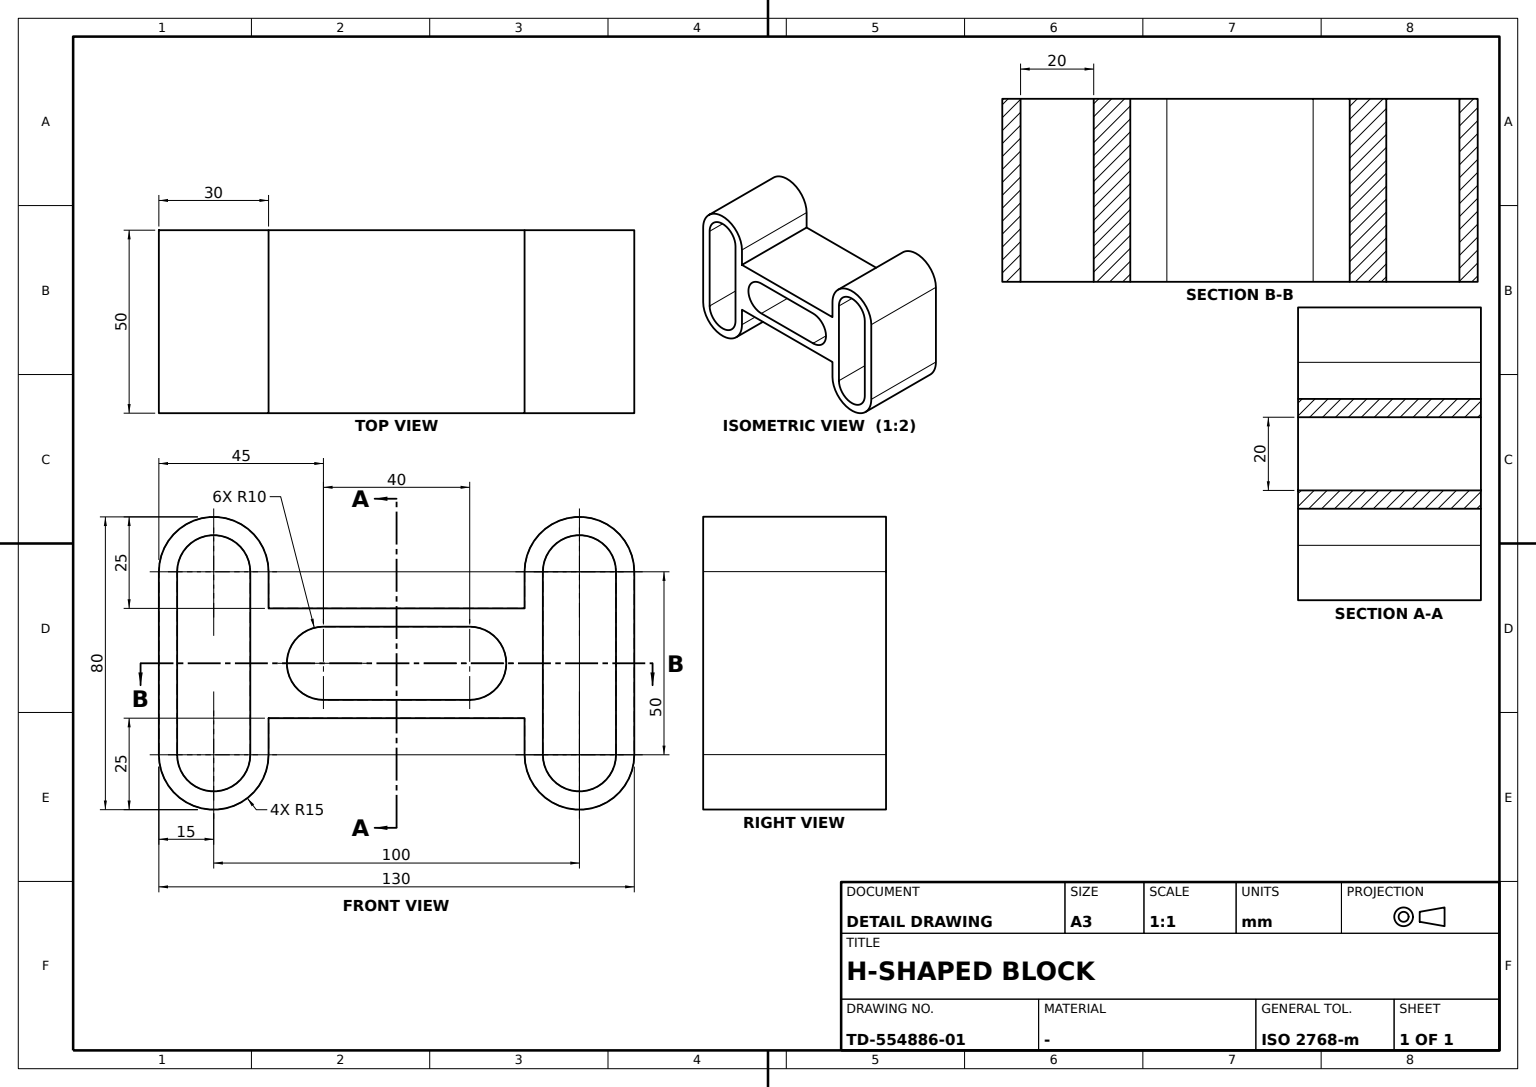
ISO-10303-21;
HEADER;
FILE_DESCRIPTION((''),'2;1');
FILE_NAME('','',(''),(''),'','','');
FILE_SCHEMA(('AUTOMOTIVE_DESIGN'));
ENDSEC;
DATA;
#1=APPLICATION_CONTEXT('');
#2=PRODUCT_CONTEXT('',#1,'mechanical');
#3=PRODUCT('','','',(#2));
#4=PRODUCT_DEFINITION_FORMATION('','',#3);
#5=PRODUCT_DEFINITION_CONTEXT('',#1,'design');
#6=PRODUCT_DEFINITION('','',#4,#5);
#7=PRODUCT_DEFINITION_SHAPE('','',#6);
#8=(LENGTH_UNIT()NAMED_UNIT(*)SI_UNIT(.MILLI.,.METRE.));
#9=(NAMED_UNIT(*)PLANE_ANGLE_UNIT()SI_UNIT($,.RADIAN.));
#10=(NAMED_UNIT(*)SI_UNIT($,.STERADIAN.)SOLID_ANGLE_UNIT());
#11=UNCERTAINTY_MEASURE_WITH_UNIT(LENGTH_MEASURE(1.E-05),#8,'distance_accuracy_value','');
#12=(GEOMETRIC_REPRESENTATION_CONTEXT(3)GLOBAL_UNCERTAINTY_ASSIGNED_CONTEXT((#11))GLOBAL_UNIT_ASSIGNED_CONTEXT((#8,#9,#10))REPRESENTATION_CONTEXT('',''));
#13=CARTESIAN_POINT('',(-25.,30.,0.));
#14=VERTEX_POINT('',#13);
#15=CARTESIAN_POINT('',(-25.,20.,10.));
#16=VERTEX_POINT('',#15);
#17=CARTESIAN_POINT('',(-25.,20.,0.));
#18=DIRECTION('',(1.,0.,0.));
#19=DIRECTION('',(0.,1.,0.));
#20=AXIS2_PLACEMENT_3D('',#17,#18,#19);
#21=CIRCLE('',#20,10.);
#22=EDGE_CURVE('',#14,#16,#21,.T.);
#23=ORIENTED_EDGE('',*,*,#22,.F.);
#24=CARTESIAN_POINT('',(25.,30.,0.));
#25=VERTEX_POINT('',#24);
#26=CARTESIAN_POINT('',(0.,30.,0.));
#27=DIRECTION('',(-1.,0.,0.));
#28=VECTOR('',#27,1000.);
#29=LINE('',#26,#28);
#30=EDGE_CURVE('',#25,#14,#29,.T.);
#31=ORIENTED_EDGE('',*,*,#30,.F.);
#32=CARTESIAN_POINT('',(25.,20.,10.));
#33=VERTEX_POINT('',#32);
#34=CARTESIAN_POINT('',(25.,20.,0.));
#35=AXIS2_PLACEMENT_3D('',#34,#18,#19);
#36=CIRCLE('',#35,10.);
#37=EDGE_CURVE('',#25,#33,#36,.T.);
#38=ORIENTED_EDGE('',*,*,#37,.T.);
#39=CARTESIAN_POINT('',(0.,20.,10.));
#40=LINE('',#39,#28);
#41=EDGE_CURVE('',#33,#16,#40,.T.);
#42=ORIENTED_EDGE('',*,*,#41,.T.);
#43=EDGE_LOOP('',(#23,#31,#38,#42));
#44=FACE_OUTER_BOUND('',#43,.T.);
#45=CARTESIAN_POINT('',(0.,20.,0.));
#46=AXIS2_PLACEMENT_3D('',#45,#27,#19);
#47=CYLINDRICAL_SURFACE('',#46,10.);
#48=ADVANCED_FACE('',(#44),#47,.F.);
#49=CARTESIAN_POINT('',(-25.,-35.,15.));
#50=VERTEX_POINT('',#49);
#51=CARTESIAN_POINT('',(25.,-35.,15.));
#52=VERTEX_POINT('',#51);
#53=CARTESIAN_POINT('',(0.,-35.,15.));
#54=VECTOR('',#18,1000.);
#55=LINE('',#53,#54);
#56=EDGE_CURVE('',#50,#52,#55,.T.);
#57=ORIENTED_EDGE('',*,*,#56,.T.);
#58=CARTESIAN_POINT('',(25.,35.,15.));
#59=VERTEX_POINT('',#58);
#60=CARTESIAN_POINT('',(25.,0.,15.));
#61=DIRECTION('',(0.,-1.,0.));
#62=VECTOR('',#61,1000.);
#63=LINE('',#60,#62);
#64=EDGE_CURVE('',#59,#52,#63,.T.);
#65=ORIENTED_EDGE('',*,*,#64,.F.);
#66=CARTESIAN_POINT('',(-25.,35.,15.));
#67=VERTEX_POINT('',#66);
#68=CARTESIAN_POINT('',(0.,35.,15.));
#69=LINE('',#68,#54);
#70=EDGE_CURVE('',#67,#59,#69,.T.);
#71=ORIENTED_EDGE('',*,*,#70,.F.);
#72=CARTESIAN_POINT('',(-25.,0.,15.));
#73=LINE('',#72,#62);
#74=EDGE_CURVE('',#67,#50,#73,.T.);
#75=ORIENTED_EDGE('',*,*,#74,.T.);
#76=EDGE_LOOP('',(#57,#65,#71,#75));
#77=FACE_OUTER_BOUND('',#76,.T.);
#78=DIRECTION('',(0.,0.,-1.));
#79=AXIS2_PLACEMENT_3D('',#53,#78,#19);
#80=PLANE('',#79);
#81=ADVANCED_FACE('',(#77),#80,.F.);
#82=CARTESIAN_POINT('',(25.,-20.,10.));
#83=VERTEX_POINT('',#82);
#84=CARTESIAN_POINT('',(25.,0.,10.));
#85=LINE('',#84,#62);
#86=EDGE_CURVE('',#33,#83,#85,.T.);
#87=ORIENTED_EDGE('',*,*,#86,.T.);
#88=CARTESIAN_POINT('',(-25.,-20.,10.));
#89=VERTEX_POINT('',#88);
#90=CARTESIAN_POINT('',(0.,-20.,10.));
#91=LINE('',#90,#28);
#92=EDGE_CURVE('',#83,#89,#91,.T.);
#93=ORIENTED_EDGE('',*,*,#92,.T.);
#94=CARTESIAN_POINT('',(-25.,0.,10.));
#95=LINE('',#94,#62);
#96=EDGE_CURVE('',#16,#89,#95,.T.);
#97=ORIENTED_EDGE('',*,*,#96,.F.);
#98=ORIENTED_EDGE('',*,*,#41,.F.);
#99=EDGE_LOOP('',(#87,#93,#97,#98));
#100=FACE_OUTER_BOUND('',#99,.T.);
#101=DIRECTION('',(0.,0.,1.));
#102=AXIS2_PLACEMENT_3D('',#90,#101,#19);
#103=PLANE('',#102);
#104=ADVANCED_FACE('',(#100),#103,.F.);
#105=CARTESIAN_POINT('',(25.,-20.,-10.));
#106=VERTEX_POINT('',#105);
#107=CARTESIAN_POINT('',(25.,20.,-10.));
#108=VERTEX_POINT('',#107);
#109=CARTESIAN_POINT('',(25.,0.,-10.));
#110=VECTOR('',#19,1000.);
#111=LINE('',#109,#110);
#112=EDGE_CURVE('',#106,#108,#111,.T.);
#113=ORIENTED_EDGE('',*,*,#112,.T.);
#114=CARTESIAN_POINT('',(-25.,20.,-10.));
#115=VERTEX_POINT('',#114);
#116=CARTESIAN_POINT('',(0.,20.,-10.));
#117=LINE('',#116,#28);
#118=EDGE_CURVE('',#108,#115,#117,.T.);
#119=ORIENTED_EDGE('',*,*,#118,.T.);
#120=CARTESIAN_POINT('',(-25.,-20.,-10.));
#121=VERTEX_POINT('',#120);
#122=CARTESIAN_POINT('',(-25.,0.,-10.));
#123=LINE('',#122,#110);
#124=EDGE_CURVE('',#121,#115,#123,.T.);
#125=ORIENTED_EDGE('',*,*,#124,.F.);
#126=CARTESIAN_POINT('',(0.,-20.,-10.));
#127=LINE('',#126,#28);
#128=EDGE_CURVE('',#106,#121,#127,.T.);
#129=ORIENTED_EDGE('',*,*,#128,.F.);
#130=EDGE_LOOP('',(#113,#119,#125,#129));
#131=FACE_OUTER_BOUND('',#130,.T.);
#132=AXIS2_PLACEMENT_3D('',#116,#78,#61);
#133=PLANE('',#132);
#134=ADVANCED_FACE('',(#131),#133,.F.);
#135=CARTESIAN_POINT('',(25.,65.,25.));
#136=VERTEX_POINT('',#135);
#137=CARTESIAN_POINT('',(25.,35.,25.));
#138=VERTEX_POINT('',#137);
#139=CARTESIAN_POINT('',(25.,50.,25.));
#140=AXIS2_PLACEMENT_3D('',#139,#18,#19);
#141=CIRCLE('',#140,15.);
#142=EDGE_CURVE('',#136,#138,#141,.T.);
#143=ORIENTED_EDGE('',*,*,#142,.F.);
#144=CARTESIAN_POINT('',(-25.,65.,25.));
#145=VERTEX_POINT('',#144);
#146=CARTESIAN_POINT('',(0.,65.,25.));
#147=LINE('',#146,#54);
#148=EDGE_CURVE('',#145,#136,#147,.T.);
#149=ORIENTED_EDGE('',*,*,#148,.F.);
#150=CARTESIAN_POINT('',(-25.,35.,25.));
#151=VERTEX_POINT('',#150);
#152=CARTESIAN_POINT('',(-25.,50.,25.));
#153=AXIS2_PLACEMENT_3D('',#152,#18,#19);
#154=CIRCLE('',#153,15.);
#155=EDGE_CURVE('',#145,#151,#154,.T.);
#156=ORIENTED_EDGE('',*,*,#155,.T.);
#157=CARTESIAN_POINT('',(0.,35.,25.));
#158=LINE('',#157,#54);
#159=EDGE_CURVE('',#151,#138,#158,.T.);
#160=ORIENTED_EDGE('',*,*,#159,.T.);
#161=EDGE_LOOP('',(#143,#149,#156,#160));
#162=FACE_OUTER_BOUND('',#161,.T.);
#163=CARTESIAN_POINT('',(0.,50.,25.));
#164=AXIS2_PLACEMENT_3D('',#163,#27,#19);
#165=CYLINDRICAL_SURFACE('',#164,15.);
#166=ADVANCED_FACE('',(#162),#165,.T.);
#167=CARTESIAN_POINT('',(-25.,35.,-15.));
#168=VERTEX_POINT('',#167);
#169=CARTESIAN_POINT('',(25.,35.,-15.));
#170=VERTEX_POINT('',#169);
#171=CARTESIAN_POINT('',(0.,35.,-15.));
#172=LINE('',#171,#54);
#173=EDGE_CURVE('',#168,#170,#172,.T.);
#174=ORIENTED_EDGE('',*,*,#173,.F.);
#175=CARTESIAN_POINT('',(-25.,35.,-25.));
#176=VERTEX_POINT('',#175);
#177=CARTESIAN_POINT('',(-25.,35.,-20.));
#178=VECTOR('',#78,1000.);
#179=LINE('',#177,#178);
#180=EDGE_CURVE('',#168,#176,#179,.T.);
#181=ORIENTED_EDGE('',*,*,#180,.T.);
#182=CARTESIAN_POINT('',(25.,35.,-25.));
#183=VERTEX_POINT('',#182);
#184=CARTESIAN_POINT('',(0.,35.,-25.));
#185=LINE('',#184,#54);
#186=EDGE_CURVE('',#176,#183,#185,.T.);
#187=ORIENTED_EDGE('',*,*,#186,.T.);
#188=CARTESIAN_POINT('',(25.,35.,-20.));
#189=LINE('',#188,#178);
#190=EDGE_CURVE('',#170,#183,#189,.T.);
#191=ORIENTED_EDGE('',*,*,#190,.F.);
#192=EDGE_LOOP('',(#174,#181,#187,#191));
#193=FACE_OUTER_BOUND('',#192,.T.);
#194=AXIS2_PLACEMENT_3D('',#171,#61,#78);
#195=PLANE('',#194);
#196=ADVANCED_FACE('',(#193),#195,.T.);
#197=CARTESIAN_POINT('',(25.,-35.,-25.));
#198=VERTEX_POINT('',#197);
#199=CARTESIAN_POINT('',(25.,-35.,-15.));
#200=VERTEX_POINT('',#199);
#201=CARTESIAN_POINT('',(25.,-35.,-20.));
#202=VECTOR('',#101,1000.);
#203=LINE('',#201,#202);
#204=EDGE_CURVE('',#198,#200,#203,.T.);
#205=ORIENTED_EDGE('',*,*,#204,.F.);
#206=CARTESIAN_POINT('',(-25.,-35.,-25.));
#207=VERTEX_POINT('',#206);
#208=CARTESIAN_POINT('',(0.,-35.,-25.));
#209=LINE('',#208,#54);
#210=EDGE_CURVE('',#207,#198,#209,.T.);
#211=ORIENTED_EDGE('',*,*,#210,.F.);
#212=CARTESIAN_POINT('',(-25.,-35.,-15.));
#213=VERTEX_POINT('',#212);
#214=CARTESIAN_POINT('',(-25.,-35.,-20.));
#215=LINE('',#214,#202);
#216=EDGE_CURVE('',#207,#213,#215,.T.);
#217=ORIENTED_EDGE('',*,*,#216,.T.);
#218=CARTESIAN_POINT('',(0.,-35.,-15.));
#219=LINE('',#218,#54);
#220=EDGE_CURVE('',#213,#200,#219,.T.);
#221=ORIENTED_EDGE('',*,*,#220,.T.);
#222=EDGE_LOOP('',(#205,#211,#217,#221));
#223=FACE_OUTER_BOUND('',#222,.T.);
#224=AXIS2_PLACEMENT_3D('',#53,#19,#101);
#225=PLANE('',#224);
#226=ADVANCED_FACE('',(#223),#225,.T.);
#227=CARTESIAN_POINT('',(25.,65.,-25.));
#228=VERTEX_POINT('',#227);
#229=CARTESIAN_POINT('',(25.,50.,-25.));
#230=AXIS2_PLACEMENT_3D('',#229,#18,#19);
#231=CIRCLE('',#230,15.);
#232=EDGE_CURVE('',#183,#228,#231,.T.);
#233=ORIENTED_EDGE('',*,*,#232,.F.);
#234=ORIENTED_EDGE('',*,*,#186,.F.);
#235=CARTESIAN_POINT('',(-25.,65.,-25.));
#236=VERTEX_POINT('',#235);
#237=CARTESIAN_POINT('',(-25.,50.,-25.));
#238=AXIS2_PLACEMENT_3D('',#237,#18,#19);
#239=CIRCLE('',#238,15.);
#240=EDGE_CURVE('',#176,#236,#239,.T.);
#241=ORIENTED_EDGE('',*,*,#240,.T.);
#242=CARTESIAN_POINT('',(0.,65.,-25.));
#243=LINE('',#242,#54);
#244=EDGE_CURVE('',#236,#228,#243,.T.);
#245=ORIENTED_EDGE('',*,*,#244,.T.);
#246=EDGE_LOOP('',(#233,#234,#241,#245));
#247=FACE_OUTER_BOUND('',#246,.T.);
#248=CARTESIAN_POINT('',(0.,50.,-25.));
#249=AXIS2_PLACEMENT_3D('',#248,#27,#19);
#250=CYLINDRICAL_SURFACE('',#249,15.);
#251=ADVANCED_FACE('',(#247),#250,.T.);
#252=CARTESIAN_POINT('',(25.,-60.,25.));
#253=VERTEX_POINT('',#252);
#254=CARTESIAN_POINT('',(-25.,-60.,25.));
#255=VERTEX_POINT('',#254);
#256=CARTESIAN_POINT('',(0.,-60.,25.));
#257=LINE('',#256,#28);
#258=EDGE_CURVE('',#253,#255,#257,.T.);
#259=ORIENTED_EDGE('',*,*,#258,.T.);
#260=CARTESIAN_POINT('',(-25.,-40.,25.));
#261=VERTEX_POINT('',#260);
#262=CARTESIAN_POINT('',(-25.,-50.,25.));
#263=AXIS2_PLACEMENT_3D('',#262,#18,#19);
#264=CIRCLE('',#263,10.);
#265=EDGE_CURVE('',#261,#255,#264,.T.);
#266=ORIENTED_EDGE('',*,*,#265,.F.);
#267=CARTESIAN_POINT('',(25.,-40.,25.));
#268=VERTEX_POINT('',#267);
#269=CARTESIAN_POINT('',(0.,-40.,25.));
#270=LINE('',#269,#28);
#271=EDGE_CURVE('',#268,#261,#270,.T.);
#272=ORIENTED_EDGE('',*,*,#271,.F.);
#273=CARTESIAN_POINT('',(25.,-50.,25.));
#274=AXIS2_PLACEMENT_3D('',#273,#18,#19);
#275=CIRCLE('',#274,10.);
#276=EDGE_CURVE('',#268,#253,#275,.T.);
#277=ORIENTED_EDGE('',*,*,#276,.T.);
#278=EDGE_LOOP('',(#259,#266,#272,#277));
#279=FACE_OUTER_BOUND('',#278,.T.);
#280=CARTESIAN_POINT('',(0.,-50.,25.));
#281=AXIS2_PLACEMENT_3D('',#280,#27,#19);
#282=CYLINDRICAL_SURFACE('',#281,10.);
#283=ADVANCED_FACE('',(#279),#282,.F.);
#284=ORIENTED_EDGE('',*,*,#30,.T.);
#285=EDGE_CURVE('',#115,#14,#21,.T.);
#286=ORIENTED_EDGE('',*,*,#285,.F.);
#287=ORIENTED_EDGE('',*,*,#118,.F.);
#288=EDGE_CURVE('',#108,#25,#36,.T.);
#289=ORIENTED_EDGE('',*,*,#288,.T.);
#290=EDGE_LOOP('',(#284,#286,#287,#289));
#291=FACE_OUTER_BOUND('',#290,.T.);
#292=ADVANCED_FACE('',(#291),#47,.F.);
#293=CARTESIAN_POINT('',(-25.,65.,0.));
#294=LINE('',#293,#202);
#295=EDGE_CURVE('',#236,#145,#294,.T.);
#296=ORIENTED_EDGE('',*,*,#295,.T.);
#297=ORIENTED_EDGE('',*,*,#148,.T.);
#298=CARTESIAN_POINT('',(25.,65.,0.));
#299=LINE('',#298,#202);
#300=EDGE_CURVE('',#228,#136,#299,.T.);
#301=ORIENTED_EDGE('',*,*,#300,.F.);
#302=ORIENTED_EDGE('',*,*,#244,.F.);
#303=EDGE_LOOP('',(#296,#297,#301,#302));
#304=FACE_OUTER_BOUND('',#303,.T.);
#305=AXIS2_PLACEMENT_3D('',#146,#61,#78);
#306=PLANE('',#305);
#307=ADVANCED_FACE('',(#304),#306,.F.);
#308=CARTESIAN_POINT('',(-25.,-65.,-25.));
#309=VERTEX_POINT('',#308);
#310=CARTESIAN_POINT('',(25.,-65.,-25.));
#311=VERTEX_POINT('',#310);
#312=CARTESIAN_POINT('',(0.,-65.,-25.));
#313=LINE('',#312,#54);
#314=EDGE_CURVE('',#309,#311,#313,.T.);
#315=ORIENTED_EDGE('',*,*,#314,.T.);
#316=CARTESIAN_POINT('',(25.,-65.,25.));
#317=VERTEX_POINT('',#316);
#318=CARTESIAN_POINT('',(25.,-65.,0.));
#319=LINE('',#318,#178);
#320=EDGE_CURVE('',#317,#311,#319,.T.);
#321=ORIENTED_EDGE('',*,*,#320,.F.);
#322=CARTESIAN_POINT('',(-25.,-65.,25.));
#323=VERTEX_POINT('',#322);
#324=CARTESIAN_POINT('',(0.,-65.,25.));
#325=LINE('',#324,#54);
#326=EDGE_CURVE('',#323,#317,#325,.T.);
#327=ORIENTED_EDGE('',*,*,#326,.F.);
#328=CARTESIAN_POINT('',(-25.,-65.,0.));
#329=LINE('',#328,#178);
#330=EDGE_CURVE('',#323,#309,#329,.T.);
#331=ORIENTED_EDGE('',*,*,#330,.T.);
#332=EDGE_LOOP('',(#315,#321,#327,#331));
#333=FACE_OUTER_BOUND('',#332,.T.);
#334=AXIS2_PLACEMENT_3D('',#324,#61,#78);
#335=PLANE('',#334);
#336=ADVANCED_FACE('',(#333),#335,.T.);
#337=ORIENTED_EDGE('',*,*,#285,.T.);
#338=ORIENTED_EDGE('',*,*,#22,.T.);
#339=ORIENTED_EDGE('',*,*,#96,.T.);
#340=CARTESIAN_POINT('',(-25.,-20.,0.));
#341=AXIS2_PLACEMENT_3D('',#340,#18,#19);
#342=CIRCLE('',#341,10.);
#343=EDGE_CURVE('',#89,#121,#342,.T.);
#344=ORIENTED_EDGE('',*,*,#343,.T.);
#345=ORIENTED_EDGE('',*,*,#124,.T.);
#346=EDGE_LOOP('',(#337,#338,#339,#344,#345));
#347=FACE_BOUND('',#346,.T.);
#348=CARTESIAN_POINT('',(-25.,40.,25.));
#349=VERTEX_POINT('',#348);
#350=CARTESIAN_POINT('',(-25.,40.,-25.));
#351=VERTEX_POINT('',#350);
#352=CARTESIAN_POINT('',(-25.,40.,0.));
#353=LINE('',#352,#178);
#354=EDGE_CURVE('',#349,#351,#353,.T.);
#355=ORIENTED_EDGE('',*,*,#354,.T.);
#356=CARTESIAN_POINT('',(-25.,60.,-25.));
#357=VERTEX_POINT('',#356);
#358=CIRCLE('',#238,10.);
#359=EDGE_CURVE('',#351,#357,#358,.T.);
#360=ORIENTED_EDGE('',*,*,#359,.T.);
#361=CARTESIAN_POINT('',(-25.,60.,25.));
#362=VERTEX_POINT('',#361);
#363=CARTESIAN_POINT('',(-25.,60.,0.));
#364=LINE('',#363,#202);
#365=EDGE_CURVE('',#357,#362,#364,.T.);
#366=ORIENTED_EDGE('',*,*,#365,.T.);
#367=CIRCLE('',#153,10.);
#368=EDGE_CURVE('',#362,#349,#367,.T.);
#369=ORIENTED_EDGE('',*,*,#368,.T.);
#370=EDGE_LOOP('',(#355,#360,#366,#369));
#371=FACE_BOUND('',#370,.T.);
#372=CARTESIAN_POINT('',(-25.,-60.,-25.));
#373=VERTEX_POINT('',#372);
#374=CARTESIAN_POINT('',(-25.,-40.,-25.));
#375=VERTEX_POINT('',#374);
#376=CARTESIAN_POINT('',(-25.,-50.,-25.));
#377=AXIS2_PLACEMENT_3D('',#376,#18,#19);
#378=CIRCLE('',#377,10.);
#379=EDGE_CURVE('',#373,#375,#378,.T.);
#380=ORIENTED_EDGE('',*,*,#379,.T.);
#381=CARTESIAN_POINT('',(-25.,-40.,0.));
#382=LINE('',#381,#202);
#383=EDGE_CURVE('',#375,#261,#382,.T.);
#384=ORIENTED_EDGE('',*,*,#383,.T.);
#385=ORIENTED_EDGE('',*,*,#265,.T.);
#386=CARTESIAN_POINT('',(-25.,-60.,0.));
#387=LINE('',#386,#178);
#388=EDGE_CURVE('',#255,#373,#387,.T.);
#389=ORIENTED_EDGE('',*,*,#388,.T.);
#390=EDGE_LOOP('',(#380,#384,#385,#389));
#391=FACE_BOUND('',#390,.T.);
#392=CARTESIAN_POINT('',(-25.,-35.,25.));
#393=VERTEX_POINT('',#392);
#394=CARTESIAN_POINT('',(-25.,-35.,20.));
#395=LINE('',#394,#202);
#396=EDGE_CURVE('',#50,#393,#395,.T.);
#397=ORIENTED_EDGE('',*,*,#396,.F.);
#398=ORIENTED_EDGE('',*,*,#74,.F.);
#399=CARTESIAN_POINT('',(-25.,35.,20.));
#400=LINE('',#399,#178);
#401=EDGE_CURVE('',#151,#67,#400,.T.);
#402=ORIENTED_EDGE('',*,*,#401,.F.);
#403=ORIENTED_EDGE('',*,*,#155,.F.);
#404=ORIENTED_EDGE('',*,*,#295,.F.);
#405=ORIENTED_EDGE('',*,*,#240,.F.);
#406=ORIENTED_EDGE('',*,*,#180,.F.);
#407=CARTESIAN_POINT('',(-25.,0.,-15.));
#408=LINE('',#407,#110);
#409=EDGE_CURVE('',#213,#168,#408,.T.);
#410=ORIENTED_EDGE('',*,*,#409,.F.);
#411=ORIENTED_EDGE('',*,*,#216,.F.);
#412=CIRCLE('',#377,15.);
#413=EDGE_CURVE('',#309,#207,#412,.T.);
#414=ORIENTED_EDGE('',*,*,#413,.F.);
#415=ORIENTED_EDGE('',*,*,#330,.F.);
#416=CIRCLE('',#263,15.);
#417=EDGE_CURVE('',#393,#323,#416,.T.);
#418=ORIENTED_EDGE('',*,*,#417,.F.);
#419=EDGE_LOOP('',(#397,#398,#402,#403,#404,#405,#406,#410,#411,#414,#415,#418));
#420=FACE_OUTER_BOUND('',#419,.T.);
#421=CARTESIAN_POINT('',(-25.,0.,0.));
#422=AXIS2_PLACEMENT_3D('',#421,#18,#19);
#423=PLANE('',#422);
#424=ADVANCED_FACE('',(#347,#371,#391,#420),#423,.F.);
#425=ORIENTED_EDGE('',*,*,#379,.F.);
#426=CARTESIAN_POINT('',(25.,-60.,-25.));
#427=VERTEX_POINT('',#426);
#428=CARTESIAN_POINT('',(0.,-60.,-25.));
#429=LINE('',#428,#28);
#430=EDGE_CURVE('',#427,#373,#429,.T.);
#431=ORIENTED_EDGE('',*,*,#430,.F.);
#432=CARTESIAN_POINT('',(25.,-40.,-25.));
#433=VERTEX_POINT('',#432);
#434=CARTESIAN_POINT('',(25.,-50.,-25.));
#435=AXIS2_PLACEMENT_3D('',#434,#18,#19);
#436=CIRCLE('',#435,10.);
#437=EDGE_CURVE('',#427,#433,#436,.T.);
#438=ORIENTED_EDGE('',*,*,#437,.T.);
#439=CARTESIAN_POINT('',(0.,-40.,-25.));
#440=LINE('',#439,#28);
#441=EDGE_CURVE('',#433,#375,#440,.T.);
#442=ORIENTED_EDGE('',*,*,#441,.T.);
#443=EDGE_LOOP('',(#425,#431,#438,#442));
#444=FACE_OUTER_BOUND('',#443,.T.);
#445=CARTESIAN_POINT('',(0.,-50.,-25.));
#446=AXIS2_PLACEMENT_3D('',#445,#27,#19);
#447=CYLINDRICAL_SURFACE('',#446,10.);
#448=ADVANCED_FACE('',(#444),#447,.F.);
#449=ORIENTED_EDGE('',*,*,#430,.T.);
#450=ORIENTED_EDGE('',*,*,#388,.F.);
#451=ORIENTED_EDGE('',*,*,#258,.F.);
#452=CARTESIAN_POINT('',(25.,-60.,0.));
#453=LINE('',#452,#178);
#454=EDGE_CURVE('',#253,#427,#453,.T.);
#455=ORIENTED_EDGE('',*,*,#454,.T.);
#456=EDGE_LOOP('',(#449,#450,#451,#455));
#457=FACE_OUTER_BOUND('',#456,.T.);
#458=AXIS2_PLACEMENT_3D('',#256,#19,#78);
#459=PLANE('',#458);
#460=ADVANCED_FACE('',(#457),#459,.T.);
#461=ORIENTED_EDGE('',*,*,#437,.F.);
#462=ORIENTED_EDGE('',*,*,#454,.F.);
#463=ORIENTED_EDGE('',*,*,#276,.F.);
#464=CARTESIAN_POINT('',(25.,-40.,0.));
#465=LINE('',#464,#202);
#466=EDGE_CURVE('',#433,#268,#465,.T.);
#467=ORIENTED_EDGE('',*,*,#466,.F.);
#468=EDGE_LOOP('',(#461,#462,#463,#467));
#469=FACE_BOUND('',#468,.T.);
#470=CARTESIAN_POINT('',(25.,60.,25.));
#471=VERTEX_POINT('',#470);
#472=CARTESIAN_POINT('',(25.,40.,25.));
#473=VERTEX_POINT('',#472);
#474=CIRCLE('',#140,10.);
#475=EDGE_CURVE('',#471,#473,#474,.T.);
#476=ORIENTED_EDGE('',*,*,#475,.F.);
#477=CARTESIAN_POINT('',(25.,60.,-25.));
#478=VERTEX_POINT('',#477);
#479=CARTESIAN_POINT('',(25.,60.,0.));
#480=LINE('',#479,#202);
#481=EDGE_CURVE('',#478,#471,#480,.T.);
#482=ORIENTED_EDGE('',*,*,#481,.F.);
#483=CARTESIAN_POINT('',(25.,40.,-25.));
#484=VERTEX_POINT('',#483);
#485=CIRCLE('',#230,10.);
#486=EDGE_CURVE('',#484,#478,#485,.T.);
#487=ORIENTED_EDGE('',*,*,#486,.F.);
#488=CARTESIAN_POINT('',(25.,40.,0.));
#489=LINE('',#488,#178);
#490=EDGE_CURVE('',#473,#484,#489,.T.);
#491=ORIENTED_EDGE('',*,*,#490,.F.);
#492=EDGE_LOOP('',(#476,#482,#487,#491));
#493=FACE_BOUND('',#492,.T.);
#494=ORIENTED_EDGE('',*,*,#86,.F.);
#495=ORIENTED_EDGE('',*,*,#37,.F.);
#496=ORIENTED_EDGE('',*,*,#288,.F.);
#497=ORIENTED_EDGE('',*,*,#112,.F.);
#498=CARTESIAN_POINT('',(25.,-20.,0.));
#499=AXIS2_PLACEMENT_3D('',#498,#18,#19);
#500=CIRCLE('',#499,10.);
#501=EDGE_CURVE('',#83,#106,#500,.T.);
#502=ORIENTED_EDGE('',*,*,#501,.F.);
#503=EDGE_LOOP('',(#494,#495,#496,#497,#502));
#504=FACE_BOUND('',#503,.T.);
#505=ORIENTED_EDGE('',*,*,#64,.T.);
#506=CARTESIAN_POINT('',(25.,-35.,25.));
#507=VERTEX_POINT('',#506);
#508=CARTESIAN_POINT('',(25.,-35.,20.));
#509=LINE('',#508,#202);
#510=EDGE_CURVE('',#52,#507,#509,.T.);
#511=ORIENTED_EDGE('',*,*,#510,.T.);
#512=CIRCLE('',#274,15.);
#513=EDGE_CURVE('',#507,#317,#512,.T.);
#514=ORIENTED_EDGE('',*,*,#513,.T.);
#515=ORIENTED_EDGE('',*,*,#320,.T.);
#516=CIRCLE('',#435,15.);
#517=EDGE_CURVE('',#311,#198,#516,.T.);
#518=ORIENTED_EDGE('',*,*,#517,.T.);
#519=ORIENTED_EDGE('',*,*,#204,.T.);
#520=CARTESIAN_POINT('',(25.,0.,-15.));
#521=LINE('',#520,#110);
#522=EDGE_CURVE('',#200,#170,#521,.T.);
#523=ORIENTED_EDGE('',*,*,#522,.T.);
#524=ORIENTED_EDGE('',*,*,#190,.T.);
#525=ORIENTED_EDGE('',*,*,#232,.T.);
#526=ORIENTED_EDGE('',*,*,#300,.T.);
#527=ORIENTED_EDGE('',*,*,#142,.T.);
#528=CARTESIAN_POINT('',(25.,35.,20.));
#529=LINE('',#528,#178);
#530=EDGE_CURVE('',#138,#59,#529,.T.);
#531=ORIENTED_EDGE('',*,*,#530,.T.);
#532=EDGE_LOOP('',(#505,#511,#514,#515,#518,#519,#523,#524,#525,#526,#527,#531));
#533=FACE_OUTER_BOUND('',#532,.T.);
#534=CARTESIAN_POINT('',(25.,0.,0.));
#535=AXIS2_PLACEMENT_3D('',#534,#18,#19);
#536=PLANE('',#535);
#537=ADVANCED_FACE('',(#469,#493,#504,#533),#536,.T.);
#538=ORIENTED_EDGE('',*,*,#210,.T.);
#539=ORIENTED_EDGE('',*,*,#517,.F.);
#540=ORIENTED_EDGE('',*,*,#314,.F.);
#541=ORIENTED_EDGE('',*,*,#413,.T.);
#542=EDGE_LOOP('',(#538,#539,#540,#541));
#543=FACE_OUTER_BOUND('',#542,.T.);
#544=CYLINDRICAL_SURFACE('',#446,15.);
#545=ADVANCED_FACE('',(#543),#544,.T.);
#546=ORIENTED_EDGE('',*,*,#365,.F.);
#547=CARTESIAN_POINT('',(0.,60.,-25.));
#548=LINE('',#547,#28);
#549=EDGE_CURVE('',#478,#357,#548,.T.);
#550=ORIENTED_EDGE('',*,*,#549,.F.);
#551=ORIENTED_EDGE('',*,*,#481,.T.);
#552=CARTESIAN_POINT('',(0.,60.,25.));
#553=LINE('',#552,#28);
#554=EDGE_CURVE('',#471,#362,#553,.T.);
#555=ORIENTED_EDGE('',*,*,#554,.T.);
#556=EDGE_LOOP('',(#546,#550,#551,#555));
#557=FACE_OUTER_BOUND('',#556,.T.);
#558=AXIS2_PLACEMENT_3D('',#552,#19,#78);
#559=PLANE('',#558);
#560=ADVANCED_FACE('',(#557),#559,.F.);
#561=ORIENTED_EDGE('',*,*,#409,.T.);
#562=ORIENTED_EDGE('',*,*,#173,.T.);
#563=ORIENTED_EDGE('',*,*,#522,.F.);
#564=ORIENTED_EDGE('',*,*,#220,.F.);
#565=EDGE_LOOP('',(#561,#562,#563,#564));
#566=FACE_OUTER_BOUND('',#565,.T.);
#567=AXIS2_PLACEMENT_3D('',#171,#101,#61);
#568=PLANE('',#567);
#569=ADVANCED_FACE('',(#566),#568,.F.);
#570=CARTESIAN_POINT('',(0.,40.,25.));
#571=LINE('',#570,#28);
#572=EDGE_CURVE('',#473,#349,#571,.T.);
#573=ORIENTED_EDGE('',*,*,#572,.F.);
#574=ORIENTED_EDGE('',*,*,#490,.T.);
#575=CARTESIAN_POINT('',(0.,40.,-25.));
#576=LINE('',#575,#28);
#577=EDGE_CURVE('',#484,#351,#576,.T.);
#578=ORIENTED_EDGE('',*,*,#577,.T.);
#579=ORIENTED_EDGE('',*,*,#354,.F.);
#580=EDGE_LOOP('',(#573,#574,#578,#579));
#581=FACE_OUTER_BOUND('',#580,.T.);
#582=AXIS2_PLACEMENT_3D('',#570,#19,#78);
#583=PLANE('',#582);
#584=ADVANCED_FACE('',(#581),#583,.T.);
#585=ORIENTED_EDGE('',*,*,#343,.F.);
#586=ORIENTED_EDGE('',*,*,#92,.F.);
#587=ORIENTED_EDGE('',*,*,#501,.T.);
#588=ORIENTED_EDGE('',*,*,#128,.T.);
#589=EDGE_LOOP('',(#585,#586,#587,#588));
#590=FACE_OUTER_BOUND('',#589,.T.);
#591=CARTESIAN_POINT('',(0.,-20.,0.));
#592=AXIS2_PLACEMENT_3D('',#591,#27,#19);
#593=CYLINDRICAL_SURFACE('',#592,10.);
#594=ADVANCED_FACE('',(#590),#593,.F.);
#595=ORIENTED_EDGE('',*,*,#383,.F.);
#596=ORIENTED_EDGE('',*,*,#441,.F.);
#597=ORIENTED_EDGE('',*,*,#466,.T.);
#598=ORIENTED_EDGE('',*,*,#271,.T.);
#599=EDGE_LOOP('',(#595,#596,#597,#598));
#600=FACE_OUTER_BOUND('',#599,.T.);
#601=AXIS2_PLACEMENT_3D('',#269,#19,#78);
#602=PLANE('',#601);
#603=ADVANCED_FACE('',(#600),#602,.F.);
#604=ORIENTED_EDGE('',*,*,#56,.F.);
#605=ORIENTED_EDGE('',*,*,#396,.T.);
#606=CARTESIAN_POINT('',(0.,-35.,25.));
#607=LINE('',#606,#54);
#608=EDGE_CURVE('',#393,#507,#607,.T.);
#609=ORIENTED_EDGE('',*,*,#608,.T.);
#610=ORIENTED_EDGE('',*,*,#510,.F.);
#611=EDGE_LOOP('',(#604,#605,#609,#610));
#612=FACE_OUTER_BOUND('',#611,.T.);
#613=ADVANCED_FACE('',(#612),#225,.T.);
#614=ORIENTED_EDGE('',*,*,#159,.F.);
#615=ORIENTED_EDGE('',*,*,#401,.T.);
#616=ORIENTED_EDGE('',*,*,#70,.T.);
#617=ORIENTED_EDGE('',*,*,#530,.F.);
#618=EDGE_LOOP('',(#614,#615,#616,#617));
#619=FACE_OUTER_BOUND('',#618,.T.);
#620=ADVANCED_FACE('',(#619),#195,.T.);
#621=ORIENTED_EDGE('',*,*,#572,.T.);
#622=ORIENTED_EDGE('',*,*,#368,.F.);
#623=ORIENTED_EDGE('',*,*,#554,.F.);
#624=ORIENTED_EDGE('',*,*,#475,.T.);
#625=EDGE_LOOP('',(#621,#622,#623,#624));
#626=FACE_OUTER_BOUND('',#625,.T.);
#627=CYLINDRICAL_SURFACE('',#164,10.);
#628=ADVANCED_FACE('',(#626),#627,.F.);
#629=ORIENTED_EDGE('',*,*,#417,.T.);
#630=ORIENTED_EDGE('',*,*,#326,.T.);
#631=ORIENTED_EDGE('',*,*,#513,.F.);
#632=ORIENTED_EDGE('',*,*,#608,.F.);
#633=EDGE_LOOP('',(#629,#630,#631,#632));
#634=FACE_OUTER_BOUND('',#633,.T.);
#635=CYLINDRICAL_SURFACE('',#281,15.);
#636=ADVANCED_FACE('',(#634),#635,.T.);
#637=ORIENTED_EDGE('',*,*,#549,.T.);
#638=ORIENTED_EDGE('',*,*,#359,.F.);
#639=ORIENTED_EDGE('',*,*,#577,.F.);
#640=ORIENTED_EDGE('',*,*,#486,.T.);
#641=EDGE_LOOP('',(#637,#638,#639,#640));
#642=FACE_OUTER_BOUND('',#641,.T.);
#643=CYLINDRICAL_SURFACE('',#249,10.);
#644=ADVANCED_FACE('',(#642),#643,.F.);
#645=CLOSED_SHELL('',(#48,#81,#104,#134,#166,#196,#226,#251,#283,#292,#307,#336,#424,#448,#460,#537,#545,#560,#569,#584,#594,#603,#613,#620,#628,#636,#644));
#646=MANIFOLD_SOLID_BREP('',#645);
#647=ADVANCED_BREP_SHAPE_REPRESENTATION('',(#646),#12);
#648=SHAPE_DEFINITION_REPRESENTATION(#7,#647);
ENDSEC;
END-ISO-10303-21;
